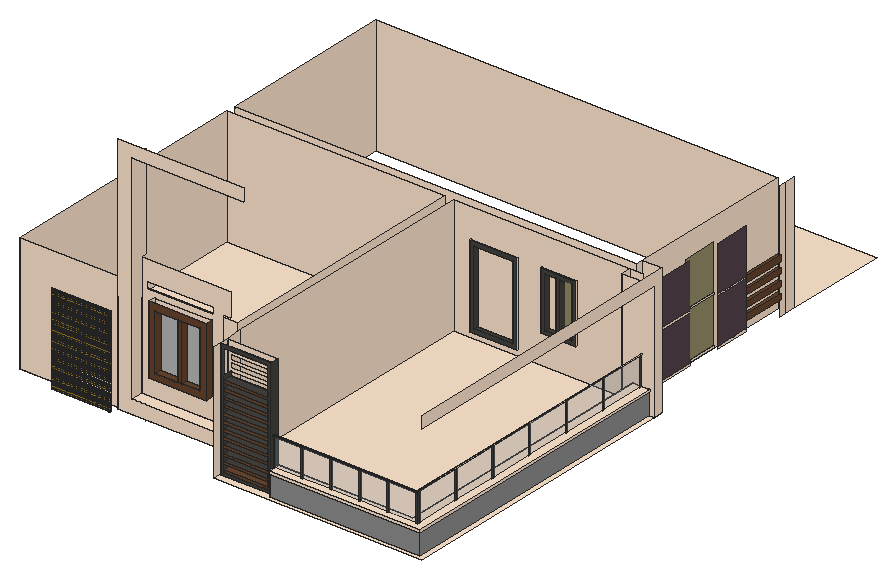
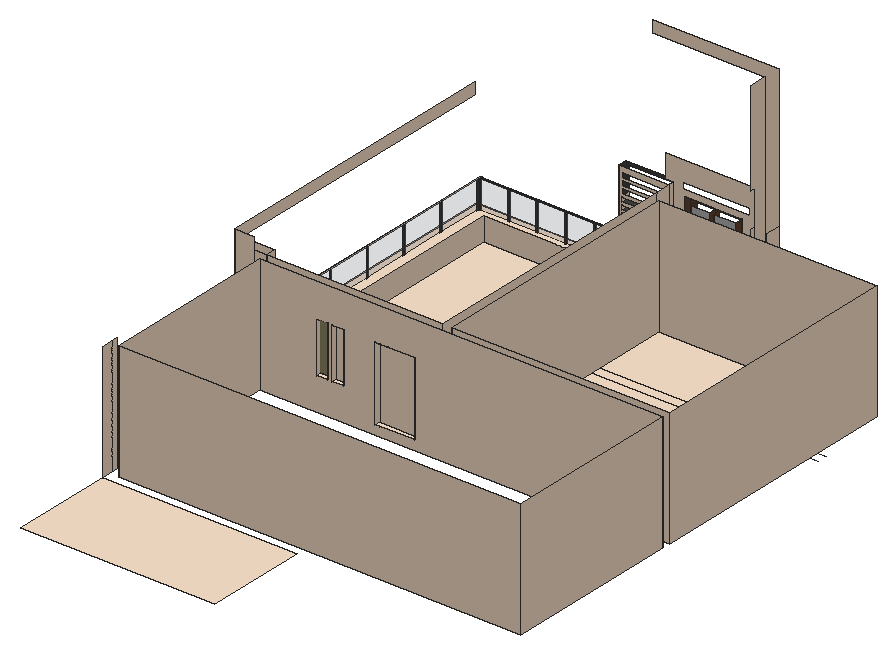
# SketchUp Ruby script. Lengths in inches.
U = 1.inch
M = Sketchup.active_model
def pt(a) = Geom::Point3d.new(a.map { |v| v * U })
def face(e, loops, mat)
  f = e.add_face(loops[0].map { |a| pt(a) })
  loops[1..].each { |l| e.add_face(l.map { |a| pt(a) }).erase! }
  f.material = f.back_material = mat if mat
  f
end
# faces: each face lists its corners as indices into pts; further lists are holes
def faces(e, pts, list, mat = nil) = list.each { |f| face(e, (f[0].is_a?(Array) ? f : [f]).map { |l| l.map { |i| pts[i] } }, mat) }
# xy, xz, yz: faces in a plane at the given z, y or x. An outline is a flat list of corners, or four numbers for a rectangle; further outlines are holes
def ring(l) = l.size == 4 ? [[l[0], l[1]], [l[2], l[1]], [l[2], l[3]], [l[0], l[3]]] : l.each_slice(2).to_a
def flat(e, list, mat, &to3) = list.each { |f| face(e, (f[0].is_a?(Array) ? f : [f]).map { |l| ring(l).map { |u, v| to3.(u, v) } }, mat) }
def xy(e, z, list, mat = nil) = flat(e, list, mat) { |x, y| [x, y, z] }
def xz(e, y, list, mat = nil) = flat(e, list, mat) { |x, z| [x, y, z] }
def yz(e, x, list, mat = nil) = flat(e, list, mat) { |y, z| [x, y, z] }
def lines(e, pts, list) = list.each { |a, b| e.add_line(pt(pts[a]), pt(pts[b])) }
# prism: a flat outline (further loops are holes) pulled along v
def prism(e, loops, v, mat = nil)
  f = face(e, loops, mat); d = Geom::Vector3d.new(v.map { |x| x * U })
  f.pushpull(f.normal.samedirection?(d) ? d.length : -d.length)
end
def box(e, o, s, mat = nil) = prism(e, [[o, [o[0] + s[0], o[1], o[2]], [o[0] + s[0], o[1] + s[1], o[2]], [o[0], o[1] + s[1], o[2]]]], [0, 0, s[2]], mat)
def at(x, y, z, deg = 0) = Geom::Transformation.translation(pt([x, y, z])) * Geom::Transformation.rotation(ORIGIN, Z_AXIS, deg.degrees)
def axes(o, x, y, z) = Geom::Transformation.new([*x, 0, *y, 0, *z, 0, *pt(o).to_a, 1])
def part(name) = M.definitions.add(name)
# library, detail: a bought-in or finely detailed component or shape, given as its bounding box
def library(name, o, s) = part(name).tap { |d| box(d.entities, o, s) }
def detail(e, o, s) = box(e.add_group.entities, o, s)
def put(e, d, t, mat = nil) = e.add_instance(d, t).tap { |i| i.material = mat if mat }
def group(e, t, mat = nil) = e.add_group.tap { |g| g.transformation = t; g.material = mat if mat }.entities
root = M.entities
M.materials.add("C01_Vanilla_Cream").color = [255, 230, 206]
M.materials.add("C04_Amber_Sunshine").color = [160, 128, 32]
M.materials.add("Carpet_04_1K").color = [85, 67, 76]
M.materials.add("Glass_Basic_01").color = [161, 173, 186]
M.materials["Glass_Basic_01"].alpha = 0.25
M.materials.add("Glass_Mirror_01").color = [147, 139, 102]
M.materials["Glass_Mirror_01"].alpha = 0.98
M.materials.add("Glass_Mirror_2").color = [185, 185, 185]
M.materials.add("M04_Stone_Frost").color = [142, 142, 142]
M.materials.add("Wood_Planks_01_1K").color = [69, 67, 63]
M.materials.add("Wood_Veneer_15_1K").color = [107, 71, 46]
M.materials.add("Wood_Veneer_15_1K1").color = [103, 69, 45]
xy(root,131.96,[[504,298.66,537,308.86]],"C01_Vanilla_Cream")
xy(root,132,[[324,2.33,537,2.33,537,308.86,531.3,308.86,531.3,6.35,378.14,6.35,378.14,18.09,515,18.09,515,308.86,324,308.86,324,36.47,324.9375,19.45],[324.9375,10.22,376.13,19.45],[93,44.86,315,119.86],[315,44.86,324,119.86],[93,119.86,315,129.77],
  [93,119.86,315,308.86],[315,119.86,324,129.77],[515,308.86,531.3,311.2],[315,506.86,513,611.86]],"C01_Vanilla_Cream")
xy(root,137.5,[[327.9375,10.22,373.13,19.45]],"Wood_Veneer_15_1K")
xy(root,138,[[342,307.36,390,308.86]],"C01_Vanilla_Cream")
xy(root,142,[[346,312.61,386,317.86]],"C01_Vanilla_Cream")
xy(root,142,[[346,307.36,386,312.61]],"Wood_Planks_01_1K")
xy(root,142.43,[[327.9375,10.22,373.13,19.45]],"Wood_Planks_01_1K")
xy(root,144.93,[[327.9375,10.22,373.13,19.45]],"Wood_Planks_01_1K")
xy(root,149.52,[[213.9,18.47,213.9,33.47,232.54,33.47,232.54,29.79,241.0625,29.79,241.0625,33.47,245.23,33.47,245.23,29.79,253.75,29.79,253.75,33.47,257.92,33.47,257.92,29.79,266.45,29.79,266.45,33.47,270.62,33.47,270.62,29.79,279.14,29.79,279.14,33.47,283.31,33.47,283.31,29.79,291.83,29.79,291.83,33.47,310.89,33.47,310.89,18.47],[228,33.47,310.89,36.47]],"C01_Vanilla_Cream")
xy(root,149.65,[[513,440.92,516,486.47]],"Wood_Veneer_15_1K1")
xy(root,149.87,[[327.9375,10.22,373.13,19.45]],"Wood_Planks_01_1K")
xy(root,152.37,[[327.9375,10.22,373.13,19.45]],"Wood_Planks_01_1K")
xy(root,153.5,[[378.14,5.35,378.14,6.35,531.3,6.35,531.3,298.66,532.3,298.66,532.3,5.35]],"C01_Vanilla_Cream")
xy(root,155.57,[[513,440.92,516,486.47]],"Wood_Veneer_15_1K1")
xy(root,156,[[378.14,5.35,532.3,5.35,532.3,298.66,531.3,298.66,531.3,308.86,515,308.86,515,18.09,378.14,18.09]],"C01_Vanilla_Cream")
xy(root,157.3,[[327.9375,10.22,373.13,19.45]],"Wood_Planks_01_1K")
xy(root,159.8,[[327.9375,10.22,373.13,19.45]],"Wood_Planks_01_1K")
xy(root,161.34,[[513,440.92,516,486.47]],"Wood_Veneer_15_1K1")
xy(root,162,[[414,307.36,450,308.86]],"C01_Vanilla_Cream")
xy(root,163.78,[[228,18.47,310.89,30.68],[228,30.68,310.89,36.47]],"C01_Vanilla_Cream")
xy(root,164.73,[[327.9375,10.22,373.13,19.45]],"Wood_Planks_01_1K")
xy(root,166,[[430,307.36,434,308.86],[418,312.61,430,317.86],[434,313.36,446,317.86]],"C01_Vanilla_Cream")
xy(root,166,[[418,307.36,430,312.61],[434,307.36,446,313.36]],"Wood_Planks_01_1K")
xy(root,167.23,[[327.9375,10.22,373.13,19.45]],"Wood_Planks_01_1K")
xy(root,167.26,[[513,440.92,516,486.47]],"Wood_Veneer_15_1K1")
xy(root,172.17,[[327.9375,10.22,373.13,19.45]],"Wood_Planks_01_1K")
xy(root,173.03,[[513,440.92,516,486.47]],"Wood_Veneer_15_1K1")
xy(root,174.67,[[327.9375,10.22,373.13,19.45]],"Wood_Planks_01_1K")
xy(root,178.95,[[513,440.92,516,486.47]],"Wood_Veneer_15_1K1")
xy(root,179.6,[[327.9375,10.22,373.13,19.45]],"Wood_Planks_01_1K")
xy(root,182.1,[[327.9375,10.22,373.13,19.45]],"Wood_Planks_01_1K")
xy(root,184.72,[[513,440.86,516,486.47]],"Wood_Veneer_15_1K1")
xy(root,184.76,[[241.3,23.62,299.94,30.68]],"Wood_Veneer_15_1K1")
xy(root,184.97,[[376.13,11.76,524.58,12.63],[523.92,12.63,524.58,298.46]],"Wood_Planks_01_1K")
xy(root,185.73,[[376.13,11.76,524.58,11.76,524.58,298.46,523.92,298.46,523.92,12.63,376.13,12.63]],"C01_Vanilla_Cream")
xy(root,187.03,[[327.9375,10.22,373.13,19.45]],"Wood_Planks_01_1K")
xy(root,189.53,[[327.9375,10.22,373.13,19.45]],"Wood_Planks_01_1K")
xy(root,190.64,[[513,440.86,516,486.47]],"Wood_Veneer_15_1K1")
xy(root,191.2,[[247.74,23.62,270.62,30.68],[274.62,23.62,293.5,30.68]],"Wood_Veneer_15_1K1")
xy(root,194.47,[[327.9375,10.22,373.13,19.45]],"Wood_Planks_01_1K")
xy(root,196.97,[[327.9375,10.22,373.13,19.45]],"Wood_Planks_01_1K")
xy(root,201.9,[[327.9375,10.22,373.13,19.45]],"Wood_Planks_01_1K")
xy(root,204.4,[[327.9375,10.22,373.13,19.45]],"Wood_Planks_01_1K")
xy(root,209.33,[[327.9375,10.22,373.13,19.45]],"Wood_Planks_01_1K")
xy(root,211.83,[[327.9375,10.22,373.13,19.45]],"Wood_Planks_01_1K")
xy(root,216.77,[[327.9375,10.22,373.13,19.45]],"Wood_Planks_01_1K")
xy(root,218,[[346,312.61,386,317.86],[418,312.61,430,317.86],[434,313.36,446,317.86]],"C01_Vanilla_Cream")
xy(root,218,[[346,307.36,386,312.61],[418,307.36,430,312.61],[434,307.36,446,313.36]],"Wood_Planks_01_1K")
xy(root,219.27,[[327.9375,10.22,373.13,19.45]],"Wood_Planks_01_1K")
xy(root,222,[[342,307.36,390,308.86],[414,307.36,450,308.86]],"C01_Vanilla_Cream")
xz(root,5.35,[[378.14,153.5,532.3,156]],"C01_Vanilla_Cream")
xz(root,6.35,[[378.14,132,531.3,153.5]],"M04_Stone_Frost")
xz(root,10.22,[[[324.9375,132,376.13,252],[327.9375,135,373.13,249]]],"Wood_Planks_01_1K")
xz(root,10.22,[[327.9375,135,373.13,137.5],[327.9375,142.43,373.13,144.93],[327.9375,149.87,373.13,152.37],[327.9375,157.3,373.13,159.8],[327.9375,164.73,373.13,167.23],
  [327.9375,172.17,373.13,174.67],[327.9375,179.6,373.13,182.1],[327.9375,187.03,373.13,189.53],[327.9375,194.47,373.13,196.97],[327.9375,201.9,373.13,204.4],
  [327.9375,209.33,373.13,211.83],[327.9375,216.77,373.13,219.27]],"Wood_Veneer_15_1K")
xz(root,11.76,[[376.13,184.97,524.58,185.73]],"C01_Vanilla_Cream")
xz(root,12.63,[[376.13,184.97,523.92,185.73]],"C01_Vanilla_Cream")
xz(root,12.63,[[378.13,156,405.42,184.97],[407.42,156,434.71,184.97],[436.71,156,464,184.97],[466,156,493.29,184.97],[495.29,156,522.58,184.97]],"Glass_Basic_01")
xz(root,12.63,[[376.13,156,378.13,184.97],[405.42,156,407.42,184.97],[434.71,156,436.71,184.97],[464,156,466,184.97],[493.29,156,495.29,184.97],
  [522.58,156,524.58,184.97]],"Wood_Planks_01_1K")
xz(root,18.09,[[378.14,132,515,156]],"C01_Vanilla_Cream")
xz(root,18.47,[[213.9,149.52,310.89,149.52,310.89,163.78,228,163.78,228,384,342,384,342,396,213.9,396]],"C01_Vanilla_Cream")
xz(root,19.45,[[[324.9375,132,376.13,252],[327.9375,241.57,373.13,246.5],[327.9375,226.7,373.13,231.63],[327.9375,211.83,373.13,216.77],[327.9375,196.97,373.13,201.9],[327.9375,189.53,373.13,194.47],[327.9375,167.23,373.13,172.17],[327.9375,159.8,373.13,164.73],[327.9375,137.5,373.13,142.43],[327.9375,234.13,373.13,239.07],[327.9375,219.27,373.13,224.2],[327.9375,204.4,373.13,209.33],[327.9375,182.1,373.13,187.03],[327.9375,174.67,373.13,179.6],[327.9375,152.37,373.13,157.3],[327.9375,144.93,373.13,149.87]]],"C01_Vanilla_Cream")
xz(root,23.62,[[[241.3,184.76,299.94,255.2],[247.74,191.2,293.5,248.75]],[270.62,191.2,274.62,248.75]],"Wood_Veneer_15_1K1")
xz(root,30.68,[[[228,163.78,310.89,163.78,310.89,264,319.15,264,319.15,288,228,288],[241.3,184.76,299.94,255.2],[233.27,260.77,301.99,267.91]]],"C01_Vanilla_Cream")
xz(root,30.68,[[247.74,191.2,270.62,248.75],[274.62,191.2,293.5,248.75]],"Glass_Mirror_2")
xz(root,33.47,[[232.54,147.41,241.0625,149.52],[245.23,147.41,253.75,149.52],[257.92,147.41,266.45,149.52],[270.62,147.41,279.14,149.52],[283.31,147.41,291.83,149.52]],"C01_Vanilla_Cream")
xz(root,36.47,[[132,131.07,192,131.41],[132,132.72,192,133.07],[132,134.37,192,134.72],[132,136.02,192,136.37],[132,137.67,192,138.02],
  [132,139.32,192,139.67],[132,140.98,192,141.32],[132,142.63,192,142.98],[132,144.28,192,144.63],[132,145.93,192,146.28],
  [132,147.58,192,147.93],[132,147.93,192,149.24],[132,149.24,192,149.58],[132,150.89,192,151.24],[132,152.54,192,152.89],
  [132,154.19,192,154.54],[132,155.84,192,156.19],[132,156.19,192,157.5],[132,157.5,192,157.84],[132,159.15,192,159.5],
  [132,160.8,192,161.15],[132,162.45,192,162.8],[132,164.1,192,164.45],[132,165.75,192,166.1],[132,167.41,192,167.75],
  [132,169.06,192,169.41],[132,170.71,192,171.06],[132,172.36,192,172.71],[132,174.01,192,174.36],[132,175.67,192,176.01],
  [132,177.32,192,177.67],[132,178.97,192,179.32],[132,180.62,192,180.97],[132,182.27,192,182.62],[132,183.93,192,184.27],
  [132,185.58,192,185.93],[132,187.23,192,187.58],[132,188.88,192,189.23],[132,190.53,192,190.88],[132,192.18,192,192.53],
  [132,193.84,192,194.18],[132,195.49,192,195.84],[132,197.14,192,197.49],[132,198.79,192,199.14],[132,200.44,192,200.79],
  [132,202.1,192,202.44],[132,203.75,192,204.1],[132,205.4,192,205.75],[132,207.05,192,207.4],[132,208.7,192,209.05],
  [132,210.36,192,210.7],[132,212.01,192,212.36],[132,213.66,192,214.01],[132,215.3125,192,215.66],[132,216.96,192,217.3125],
  [132,218.61,192,218.96],[132,220.27,192,220.61],[132,221.92,192,222.27]],"C01_Vanilla_Cream")
xz(root,36.47,[[132,131.41,192,132.72],[132,133.07,192,134.37],[132,134.72,192,136.02],[132,136.37,192,137.67],[132,138.02,192,139.32],
  [132,139.67,192,140.98],[132,141.32,192,142.63],[132,142.98,192,144.28],[132,144.63,192,145.93],[132,146.28,192,147.58],
  [132,149.58,192,150.89],[132,151.24,192,152.54],[132,152.89,192,154.19],[132,154.54,192,155.84],[132,157.84,192,159.15],
  [132,159.5,192,160.8],[132,161.15,192,162.45],[132,162.8,192,164.1],[132,164.45,192,165.75],[132,166.1,192,167.41],
  [132,167.75,192,169.06],[132,169.41,192,170.71],[132,171.06,192,172.36],[132,172.71,192,174.01],[132,174.36,192,175.67],
  [132,176.01,192,177.32],[132,177.67,192,178.97],[132,179.32,192,180.62],[132,180.97,192,182.27],[132,182.62,192,183.93],
  [132,184.27,192,185.58],[132,185.93,192,187.23],[132,187.58,192,188.88],[132,189.23,192,190.53],[132,190.88,192,192.18],
  [132,192.53,192,193.84],[132,194.18,192,195.49],[132,195.84,192,197.14],[132,197.49,192,198.79],[132,199.14,192,200.44],
  [132,200.79,192,202.1],[132,202.44,192,203.75],[132,204.1,192,205.4],[132,205.75,192,207.05],[132,207.4,192,208.7],
  [132,209.05,192,210.36],[132,210.7,192,212.01],[132,212.36,192,213.66],[132,214.01,192,215.3125],[132,215.66,192,216.96],
  [132,217.3125,192,218.61],[132,218.96,192,220.27],[132,220.61,192,221.92],[132,222.27,192,223.57]],"C04_Amber_Sunshine")
xz(root,44.86,[[93,132,315,252]],"C01_Vanilla_Cream")
xz(root,298.46,[[523.92,184.97,524.58,185.73]],"Wood_Planks_01_1K")
xz(root,298.66,[[504,131.96,537,252],[531.3,153.5,532.3,156]],"C01_Vanilla_Cream")
xz(root,307.36,[[[342,138,390,222],[346,142,386,218]],[[414,162,450,222],[418,166,418,218,430,218,430,166,434,166,434,218,446,218,446,166]]],"Wood_Planks_01_1K")
xz(root,308.86,[[504,131.96,517,132],[517,131.96,537,132],[93,132,315,252],[[324,132,504,252],[342,138,390,222],[414,162,450,222]],[504,132,504,252,517,252,517,156,515,156,515,132],
  [515,132,517,156],[517,132,531.3,156],[531.3,132,531.3,156,517,156,517,264,537,264,537,132]],"C01_Vanilla_Cream")
xz(root,312.61,[[346,142,386,218],[418,166,430,218]],"C01_Vanilla_Cream")
xz(root,313.36,[[434,166,446,218]],"Glass_Mirror_01")
xz(root,317.86,[[[93,132,504,252],[346,142,386,218],[434,166,446,218],[418,166,430,218]]],"C01_Vanilla_Cream")
xz(root,440.92,[[513,149.65,516,155.57],[513,161.34,516,167.26],[513,173.03,516,178.95]],"C01_Vanilla_Cream")
xz(root,486.47,[[513,149.65,516,155.57],[513,161.34,516,167.26],[513,173.03,516,178.95],[513,184.72,516,190.64]],"C01_Vanilla_Cream")
xz(root,497.86,[[93,132,504,252]],"C01_Vanilla_Cream")
yz(root,93,[[44.86,132,308.86,252],[317.86,132,497.86,252]],"C01_Vanilla_Cream")
yz(root,213.9,[[18.47,149.52,33.47,252]],"C01_Vanilla_Cream")
yz(root,228,[[36.13,135.59,36.47,147.41],[18.47,163.78,30.68,163.78,30.68,288,36.47,288,36.47,384,18.47,384],[30.68,163.78,36.47,252]],"C01_Vanilla_Cream")
yz(root,241.3,[[23.62,184.76,30.68,255.2]],"C01_Vanilla_Cream")
yz(root,247.74,[[23.62,191.2,30.68,248.75]],"Wood_Veneer_15_1K1")
yz(root,270.62,[[23.62,191.2,30.68,248.75]],"Wood_Veneer_15_1K1")
yz(root,274.62,[[23.62,191.2,30.68,248.75]],"Wood_Veneer_15_1K1")
yz(root,293.5,[[23.62,191.2,30.68,248.75]],"Wood_Veneer_15_1K1")
yz(root,299.94,[[23.62,184.76,30.68,255.2]],"Wood_Veneer_15_1K1")
yz(root,310.89,[[33.47,147.41,36.47,149.52]],"C01_Vanilla_Cream")
yz(root,315,[[44.86,132,308.86,252]],"C01_Vanilla_Cream")
yz(root,324,[[36.47,132,308.86,252]],"C01_Vanilla_Cream")
yz(root,324.9375,[[10.22,132,19.45,252]],"C01_Vanilla_Cream")
yz(root,327.9375,[[10.22,137.5,19.45,142.43],[10.22,144.93,19.45,149.87],[10.22,152.37,19.45,157.3],[10.22,159.8,19.45,164.73],[10.22,167.23,19.45,172.17],
  [10.22,174.67,19.45,179.6],[10.22,182.1,19.45,187.03],[10.22,189.53,19.45,194.47],[10.22,196.97,19.45,201.9],[10.22,204.4,19.45,209.33],
  [10.22,211.83,19.45,216.77],[10.22,219.27,19.45,224.2]],"Wood_Planks_01_1K")
yz(root,342,[[307.36,138,308.86,222]],"C01_Vanilla_Cream")
yz(root,346,[[312.61,142,317.86,218]],"C01_Vanilla_Cream")
yz(root,346,[[307.36,142,312.61,218]],"Wood_Planks_01_1K")
yz(root,373.13,[[10.22,137.5,19.45,142.43],[10.22,144.93,19.45,149.87],[10.22,152.37,19.45,157.3],[10.22,159.8,19.45,164.73],[10.22,167.23,19.45,172.17],
  [10.22,174.67,19.45,179.6],[10.22,182.1,19.45,187.03],[10.22,189.53,19.45,194.47],[10.22,196.97,19.45,201.9],[10.22,204.4,19.45,209.33],
  [10.22,211.83,19.45,216.77],[10.22,219.27,19.45,224.2]],"C01_Vanilla_Cream")
yz(root,376.13,[[[10.22,132,19.45,252],[11.76,184.97,12.63,185.73]]],"Wood_Planks_01_1K")
yz(root,378.14,[[6.35,132,6.35,153.5,5.35,153.5,5.35,156,18.09,156,18.09,132]],"C01_Vanilla_Cream")
yz(root,386,[[312.61,142,317.86,218]],"C01_Vanilla_Cream")
yz(root,386,[[307.36,142,312.61,218]],"Wood_Planks_01_1K")
yz(root,390,[[307.36,138,308.86,222]],"C01_Vanilla_Cream")
yz(root,414,[[307.36,162,308.86,222]],"C01_Vanilla_Cream")
yz(root,418,[[312.61,166,317.86,218]],"C01_Vanilla_Cream")
yz(root,418,[[307.36,166,312.61,218]],"Wood_Planks_01_1K")
yz(root,430,[[312.61,166,317.86,218]],"C01_Vanilla_Cream")
yz(root,430,[[307.36,166,312.61,218]],"Wood_Planks_01_1K")
yz(root,434,[[313.36,166,317.86,218]],"C01_Vanilla_Cream")
yz(root,434,[[307.36,166,313.36,218]],"Wood_Planks_01_1K")
yz(root,446,[[313.36,166,317.86,218]],"C01_Vanilla_Cream")
yz(root,446,[[307.36,166,313.36,218]],"Wood_Planks_01_1K")
yz(root,450,[[307.36,162,308.86,222]],"C01_Vanilla_Cream")
yz(root,504,[[298.66,131.96,308.86,252],[317.86,132,497.86,252]],"C01_Vanilla_Cream")
yz(root,513,[[488.83,132,494.76,252],[494.76,132,506.86,252],[368.86,140.8,404.86,142.8],[368.86,189.04,404.86,191.04]],"C01_Vanilla_Cream")
yz(root,513,[[368.86,142.8,404.86,189.04],[368.86,191.04,404.86,237.28]],"Glass_Mirror_01")
yz(root,515,[[18.09,132,308.86,156]],"C01_Vanilla_Cream")
yz(root,516,[[440.92,149.65,486.47,155.57],[440.92,161.34,486.47,167.26],[440.92,173.03,486.47,178.95],[440.86,184.72,486.47,190.64]],"Wood_Veneer_15_1K1")
yz(root,517,[[308.86,141.18,368.86,143.18],[404.86,141.18,440.86,143.18],[308.86,189.34,368.86,191.34],[404.86,189.34,440.86,191.34]],"C01_Vanilla_Cream")
yz(root,517,[[308.86,143.18,368.86,189.34],[404.86,143.18,440.86,189.34],[308.86,191.34,368.86,237.51],[404.86,191.34,440.86,237.51]],"Carpet_04_1K")
yz(root,523.92,[[12.63,184.97,298.46,185.73]],"C01_Vanilla_Cream")
yz(root,524.58,[[11.76,184.97,298.46,185.73]],"C01_Vanilla_Cream")
yz(root,524.58,[[14.63,156,59.72,184.97],[61.72,156,106.81,184.97],[108.81,156,153.9,184.97],[155.9,156,200.99,184.97],[202.99,156,248.08,184.97],
  [250.08,156,295.17,184.97]],"Glass_Basic_01")
yz(root,524.58,[[12.63,156,14.63,184.97],[59.72,156,61.72,184.97],[106.81,156,108.81,184.97],[153.9,156,155.9,184.97],[200.99,156,202.99,184.97],
  [248.08,156,250.08,184.97],[295.17,156,297.17,184.97]],"Wood_Planks_01_1K")
yz(root,531.3,[[6.35,132,308.86,132,308.86,156,298.66,156,298.66,153.5,6.35,153.5]],"M04_Stone_Frost")
yz(root,532.3,[[5.35,153.5,298.66,156]],"C01_Vanilla_Cream")
yz(root,537,[[298.66,131.96,308.86,132],[298.66,132,308.86,132,308.86,264,2.33,264,2.33,252,298.66,252]],"C01_Vanilla_Cream")
p = [[324,2.33,132],[324.9375,19.45,132],[324.9375,19.45,252],[324,2.33,252],[324,36.47,132],[324,36.47,252],
  [93,129.77,132],[84,129.77,132],[84,119.86,132],[93,119.86,132],[228,36.13,147.41],[228,33.47,147.41]]
faces(root,p,[[0,1,2,3],[1,4,5,2]],"C01_Vanilla_Cream")
lines(root,p,[[6,7],[8,9],[10,11]])
